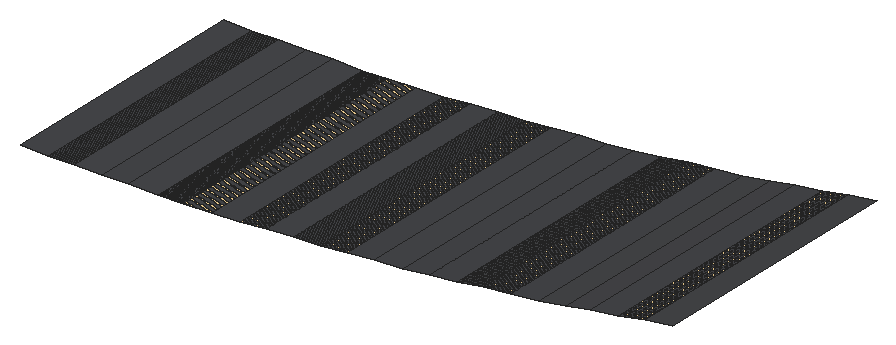
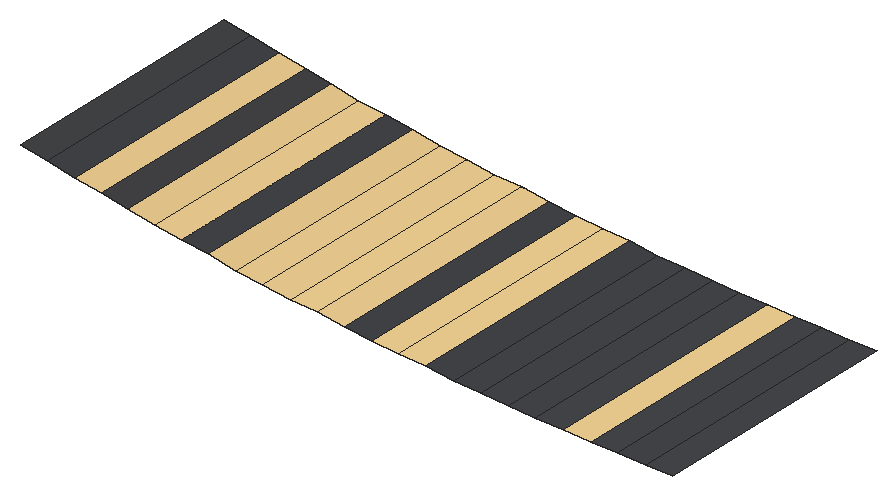
# SketchUp Ruby script. Lengths in inches.
U = 1.inch
M = Sketchup.active_model
def pt(a) = Geom::Point3d.new(a.map { |v| v * U })
def face(e, loops, mat)
  f = e.add_face(loops[0].map { |a| pt(a) })
  loops[1..].each { |l| e.add_face(l.map { |a| pt(a) }).erase! }
  f.material = f.back_material = mat if mat
  f
end
# faces: each face lists its corners as indices into pts; further lists are holes
def faces(e, pts, list, mat = nil) = list.each { |f| face(e, (f[0].is_a?(Array) ? f : [f]).map { |l| l.map { |i| pts[i] } }, mat) }
# xy, xz, yz: faces in a plane at the given z, y or x. An outline is a flat list of corners, or four numbers for a rectangle; further outlines are holes
def ring(l) = l.size == 4 ? [[l[0], l[1]], [l[2], l[1]], [l[2], l[3]], [l[0], l[3]]] : l.each_slice(2).to_a
def flat(e, list, mat, &to3) = list.each { |f| face(e, (f[0].is_a?(Array) ? f : [f]).map { |l| ring(l).map { |u, v| to3.(u, v) } }, mat) }
def xy(e, z, list, mat = nil) = flat(e, list, mat) { |x, y| [x, y, z] }
def xz(e, y, list, mat = nil) = flat(e, list, mat) { |x, z| [x, y, z] }
def yz(e, x, list, mat = nil) = flat(e, list, mat) { |y, z| [x, y, z] }
def lines(e, pts, list) = list.each { |a, b| e.add_line(pt(pts[a]), pt(pts[b])) }
# prism: a flat outline (further loops are holes) pulled along v
def prism(e, loops, v, mat = nil)
  f = face(e, loops, mat); d = Geom::Vector3d.new(v.map { |x| x * U })
  f.pushpull(f.normal.samedirection?(d) ? d.length : -d.length)
end
def box(e, o, s, mat = nil) = prism(e, [[o, [o[0] + s[0], o[1], o[2]], [o[0] + s[0], o[1] + s[1], o[2]], [o[0], o[1] + s[1], o[2]]]], [0, 0, s[2]], mat)
def at(x, y, z, deg = 0) = Geom::Transformation.translation(pt([x, y, z])) * Geom::Transformation.rotation(ORIGIN, Z_AXIS, deg.degrees)
def axes(o, x, y, z) = Geom::Transformation.new([*x, 0, *y, 0, *z, 0, *pt(o).to_a, 1])
def part(name) = M.definitions.add(name)
# library, detail: a bought-in or finely detailed component or shape, given as its bounding box
def library(name, o, s) = part(name).tap { |d| box(d.entities, o, s) }
def detail(e, o, s) = box(e.add_group.entities, o, s)
def put(e, d, t, mat = nil) = e.add_instance(d, t).tap { |i| i.material = mat if mat }
def group(e, t, mat = nil) = e.add_group.tap { |g| g.transformation = t; g.material = mat if mat }.entities
root = M.entities
M.materials.add("1432 AP 8245 TAR ROAD").color = [71, 72, 75]
M.materials.add("Outer Light").color = [251, 217, 152]
xy(root,171.29,[[537.16,95.37,537.32,96.87]],"1432 AP 8245 TAR ROAD")
xy(root,171.29,[[537.16,95.37,537.32,96.87]],"Outer Light")
xy(root,171.3,[[537.48,95.37,537.64,96.87]],"1432 AP 8245 TAR ROAD")
xy(root,171.3,[[537.48,95.37,537.64,96.87]],"Outer Light")
xy(root,171.31,[[537.8,95.37,537.97,96.87]],"1432 AP 8245 TAR ROAD")
xy(root,171.31,[[537.8,95.37,537.97,96.87]],"Outer Light")
p = [[537.32,95.37,171.29],[537.48,95.37,171.3],[537.48,96.87,171.3],[537.32,96.87,171.29],[537.32,96.87,171.29],[537.48,96.87,171.3],
  [537.48,95.37,171.3],[537.32,95.37,171.29],[537.64,95.37,171.3],[537.8,95.37,171.31],[537.8,96.87,171.31],[537.64,96.87,171.3],
  [537.64,96.87,171.3],[537.8,96.87,171.31],[537.8,95.37,171.31],[537.64,95.37,171.3],[537.97,95.37,171.31],[538.125,95.37,171.32],
  [538.125,96.87,171.32],[537.97,96.87,171.31],[537.97,96.87,171.31],[538.125,96.87,171.32],[538.125,95.37,171.32],[537.97,95.37,171.31],
  [538.29,95.37,171.33],[538.29,96.87,171.33],[538.29,96.87,171.33],[538.29,95.37,171.33],[538.45,95.37,171.34],[538.45,96.87,171.34],
  [538.45,96.87,171.34],[538.45,95.37,171.34],[538.61,95.37,171.36],[538.61,96.87,171.36],[538.61,96.87,171.36],[538.61,95.37,171.36],
  [538.77,95.37,171.37],[538.77,96.87,171.37],[538.77,96.87,171.37],[538.77,95.37,171.37],[538.93,95.37,171.38],[538.93,96.87,171.38],
  [538.93,96.87,171.38],[538.93,95.37,171.38],[539.09,95.37,171.4],[539.09,96.87,171.4],[539.09,96.87,171.4],[539.09,95.37,171.4],
  [539.25,95.37,171.42],[539.25,96.87,171.42],[539.25,96.87,171.42],[539.25,95.37,171.42],[539.41,95.37,171.43],[539.41,96.87,171.43],
  [539.41,96.87,171.43],[539.41,95.37,171.43],[539.57,95.37,171.45],[539.57,96.87,171.45],[539.57,96.87,171.45],[539.57,95.37,171.45],
  [539.73,95.37,171.47],[539.73,96.87,171.47],[539.73,96.87,171.47],[539.73,95.37,171.47],[539.89,95.37,171.5],[539.89,96.87,171.5],
  [539.89,96.87,171.5],[539.89,95.37,171.5],[540.05,95.37,171.52],[540.05,96.87,171.52],[540.05,96.87,171.52],[540.05,95.37,171.52],
  [540.21,95.37,171.54],[540.21,96.87,171.54],[540.21,96.87,171.54],[540.21,95.37,171.54],[540.37,95.37,171.57],[540.37,96.87,171.57],
  [540.37,96.87,171.57],[540.37,95.37,171.57],[540.52,95.37,171.6],[540.52,96.87,171.6],[540.52,96.87,171.6],[540.52,95.37,171.6],
  [540.68,95.37,171.625],[540.68,96.87,171.625],[540.68,96.87,171.625],[540.68,95.37,171.625],[540.84,95.37,171.66],[540.84,96.87,171.66],
  [540.84,96.87,171.66],[540.84,95.37,171.66],[541,95.37,171.6875],[541,96.87,171.6875]]
faces(root,p,[[0,1,2,3],[8,9,10,11],[16,17,18,19],[17,24,25,18],[24,28,29,25],[28,32,33,29],[32,36,37,33],[36,40,41,37],
  [40,44,45,41],[44,48,49,45],[48,52,53,49],[52,56,57,53],[56,60,61,57],[60,64,65,61],[64,68,69,65],[68,72,73,69],
  [72,76,77,73],[76,80,81,77],[80,84,85,81],[84,88,89,85],[88,92,93,89]],"1432 AP 8245 TAR ROAD")
faces(root,p,[[4,5,6,7],[12,13,14,15],[20,21,22,23],[21,26,27,22],[26,30,31,27],[30,34,35,31],[34,38,39,35],[38,42,43,39],
  [42,46,47,43],[46,50,51,47],[50,54,55,51],[54,58,59,55],[58,62,63,59],[62,66,67,63],[66,70,71,67],[70,74,75,71],
  [74,78,79,75],[78,82,83,79],[82,86,87,83],[86,90,91,87]],"Outer Light")
